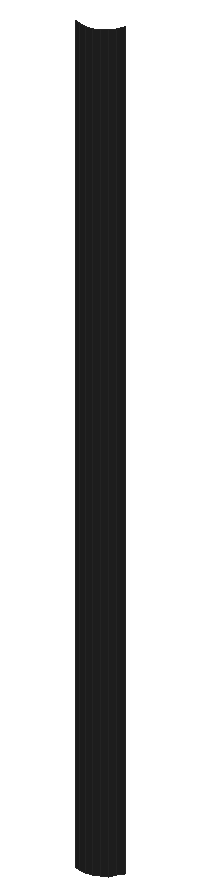
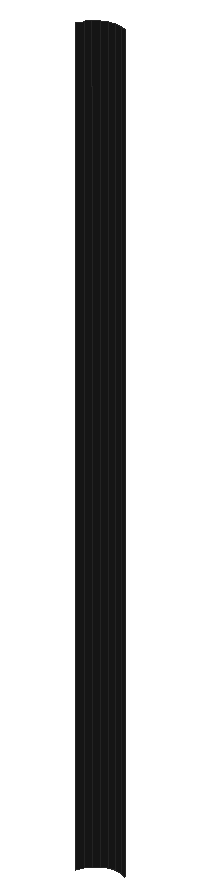
# SketchUp Ruby script. Lengths in inches.
U = 1.inch
M = Sketchup.active_model
def pt(a) = Geom::Point3d.new(a.map { |v| v * U })
def face(e, loops, mat)
  f = e.add_face(loops[0].map { |a| pt(a) })
  loops[1..].each { |l| e.add_face(l.map { |a| pt(a) }).erase! }
  f.material = f.back_material = mat if mat
  f
end
# faces: each face lists its corners as indices into pts; further lists are holes
def faces(e, pts, list, mat = nil) = list.each { |f| face(e, (f[0].is_a?(Array) ? f : [f]).map { |l| l.map { |i| pts[i] } }, mat) }
# xy, xz, yz: faces in a plane at the given z, y or x. An outline is a flat list of corners, or four numbers for a rectangle; further outlines are holes
def ring(l) = l.size == 4 ? [[l[0], l[1]], [l[2], l[1]], [l[2], l[3]], [l[0], l[3]]] : l.each_slice(2).to_a
def flat(e, list, mat, &to3) = list.each { |f| face(e, (f[0].is_a?(Array) ? f : [f]).map { |l| ring(l).map { |u, v| to3.(u, v) } }, mat) }
def xy(e, z, list, mat = nil) = flat(e, list, mat) { |x, y| [x, y, z] }
def xz(e, y, list, mat = nil) = flat(e, list, mat) { |x, z| [x, y, z] }
def yz(e, x, list, mat = nil) = flat(e, list, mat) { |y, z| [x, y, z] }
def lines(e, pts, list) = list.each { |a, b| e.add_line(pt(pts[a]), pt(pts[b])) }
# prism: a flat outline (further loops are holes) pulled along v
def prism(e, loops, v, mat = nil)
  f = face(e, loops, mat); d = Geom::Vector3d.new(v.map { |x| x * U })
  f.pushpull(f.normal.samedirection?(d) ? d.length : -d.length)
end
def box(e, o, s, mat = nil) = prism(e, [[o, [o[0] + s[0], o[1], o[2]], [o[0] + s[0], o[1] + s[1], o[2]], [o[0], o[1] + s[1], o[2]]]], [0, 0, s[2]], mat)
def at(x, y, z, deg = 0) = Geom::Transformation.translation(pt([x, y, z])) * Geom::Transformation.rotation(ORIGIN, Z_AXIS, deg.degrees)
def axes(o, x, y, z) = Geom::Transformation.new([*x, 0, *y, 0, *z, 0, *pt(o).to_a, 1])
def part(name) = M.definitions.add(name)
# library, detail: a bought-in or finely detailed component or shape, given as its bounding box
def library(name, o, s) = part(name).tap { |d| box(d.entities, o, s) }
def detail(e, o, s) = box(e.add_group.entities, o, s)
def put(e, d, t, mat = nil) = e.add_instance(d, t).tap { |i| i.material = mat if mat }
def group(e, t, mat = nil) = e.add_group.tap { |g| g.transformation = t; g.material = mat if mat }.entities
root = M.entities
M.materials.add("[0136_Charcoal]").color = [35, 35, 35]
p = [[203.05,227.61,142.6875],[203.28,227.52,142.6875],[203.28,227.52,171.43],[203.05,227.61,171.43],[203.52,227.49,142.6875],[203.52,227.49,171.43],
  [203.76,227.52,142.6875],[203.76,227.52,171.43],[203.99,227.61,142.6875],[203.99,227.61,171.43],[204.18,227.76,142.6875],[204.18,227.76,171.43],
  [204.33,227.96,142.6875],[204.33,227.96,171.43],[204.29,227.9,171.43],[204.43,228.18,142.6875],[204.43,228.18,171.43]]
faces(root,p,[[0,1,2,3],[1,4,5,2],[4,6,7,5],[6,8,9,7],[8,10,11,9],[10,12,13,14,11],[12,15,16,13]],"[0136_Charcoal]")
